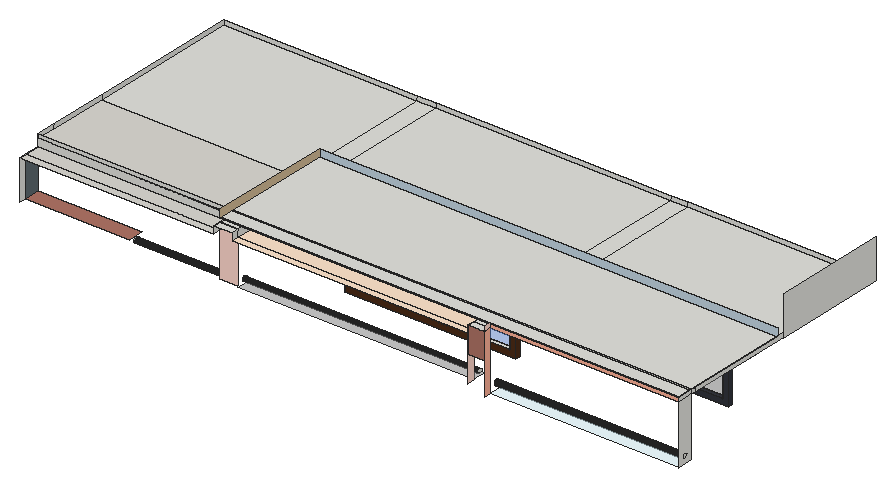
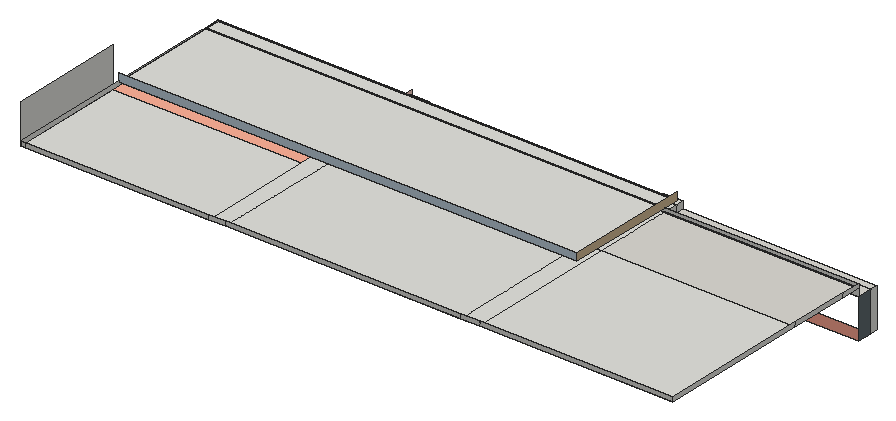
# SketchUp Ruby script. Lengths in inches.
U = 1.inch
M = Sketchup.active_model
def pt(a) = Geom::Point3d.new(a.map { |v| v * U })
def face(e, loops, mat)
  f = e.add_face(loops[0].map { |a| pt(a) })
  loops[1..].each { |l| e.add_face(l.map { |a| pt(a) }).erase! }
  f.material = f.back_material = mat if mat
  f
end
# faces: each face lists its corners as indices into pts; further lists are holes
def faces(e, pts, list, mat = nil) = list.each { |f| face(e, (f[0].is_a?(Array) ? f : [f]).map { |l| l.map { |i| pts[i] } }, mat) }
# xy, xz, yz: faces in a plane at the given z, y or x. An outline is a flat list of corners, or four numbers for a rectangle; further outlines are holes
def ring(l) = l.size == 4 ? [[l[0], l[1]], [l[2], l[1]], [l[2], l[3]], [l[0], l[3]]] : l.each_slice(2).to_a
def flat(e, list, mat, &to3) = list.each { |f| face(e, (f[0].is_a?(Array) ? f : [f]).map { |l| ring(l).map { |u, v| to3.(u, v) } }, mat) }
def xy(e, z, list, mat = nil) = flat(e, list, mat) { |x, y| [x, y, z] }
def xz(e, y, list, mat = nil) = flat(e, list, mat) { |x, z| [x, y, z] }
def yz(e, x, list, mat = nil) = flat(e, list, mat) { |y, z| [x, y, z] }
def lines(e, pts, list) = list.each { |a, b| e.add_line(pt(pts[a]), pt(pts[b])) }
# prism: a flat outline (further loops are holes) pulled along v
def prism(e, loops, v, mat = nil)
  f = face(e, loops, mat); d = Geom::Vector3d.new(v.map { |x| x * U })
  f.pushpull(f.normal.samedirection?(d) ? d.length : -d.length)
end
def box(e, o, s, mat = nil) = prism(e, [[o, [o[0] + s[0], o[1], o[2]], [o[0] + s[0], o[1] + s[1], o[2]], [o[0], o[1] + s[1], o[2]]]], [0, 0, s[2]], mat)
def at(x, y, z, deg = 0) = Geom::Transformation.translation(pt([x, y, z])) * Geom::Transformation.rotation(ORIGIN, Z_AXIS, deg.degrees)
def axes(o, x, y, z) = Geom::Transformation.new([*x, 0, *y, 0, *z, 0, *pt(o).to_a, 1])
def part(name) = M.definitions.add(name)
# library, detail: a bought-in or finely detailed component or shape, given as its bounding box
def library(name, o, s) = part(name).tap { |d| box(d.entities, o, s) }
def detail(e, o, s) = box(e.add_group.entities, o, s)
def put(e, d, t, mat = nil) = e.add_instance(d, t).tap { |i| i.material = mat if mat }
def group(e, t, mat = nil) = e.add_group.tap { |g| g.transformation = t; g.material = mat if mat }.entities
root = M.entities
M.materials.add("[Color B01]").color = [255, 216, 204]
M.materials.add("[Color B02]").color = [255, 178, 153]
M.materials.add("[Color C01]").color = [255, 229, 204]
M.materials.add("[Formica Beige]").color = [211, 187, 149]
M.materials.add("[Formica Graystone]").color = [149, 146, 135]
M.materials.add("[Formica Laminate Dark]").color = [50, 53, 60]
M.materials.add("[Formica Speckled Grey]").color = [94, 105, 111]
M.materials.add("[Stone Flagstone Ashlar]").color = [175, 116, 102]
M.materials.add("[Stone Flagstone Ashlar]1").color = [175, 116, 102]
M.materials.add("[Terrazzo Light Blue]").color = [196, 214, 227]
M.materials.add("[Terrazzo Tile Light]").color = [219, 217, 210]
M.materials.add("[Translucent Glass Blue]").color = [100, 149, 237]
M.materials["[Translucent Glass Blue]"].alpha = 0.5
M.materials.add("[Translucent Glass Gray]").color = [128, 128, 128]
M.materials["[Translucent Glass Gray]"].alpha = 0.5
M.materials.add("[Translucent Glass Safety]").color = [204, 235, 244]
M.materials["[Translucent Glass Safety]"].alpha = 0.5
M.materials.add("[Wood Veneer 01]").color = [76, 44, 23]
xy(root,2142.09,[[1358.7,1144.55,1824.89,1156.55]])
xy(root,2155.2,[[2073.08,1246.05,2321.89,1258.05]])
xy(root,2158.13,[[1374.73,1144.55,1482.83,1156.55],[1499.58,1144.55,1598.96,1156.55],[1615.7,1144.55,1695.53,1156.55],[1712.28,1144.55,1808.85,1156.55]])
xy(root,2169.37,[[2087.25,1246.05,2188.13,1258.05],[2208.5,1246.05,2307.73,1258.05]],"[Formica Laminate Dark]")
xy(root,2209.0625,[[1950.59,899.87,2463.34,941.93]],"[Translucent Glass Safety]")
xy(root,2226.5,[[1263.92,899.87,1905.54,941.93]],"[Translucent Glass Gray]")
xy(root,2228,[[1110.56,919.11,1111.89,919.29,1113.12,919.8,1114.18,920.61,1115,921.68,1115.51,922.91,1115.68,924.24,1115.51,925.57,1115,926.8,1114.18,927.86,1113.12,928.68,1111.89,929.1875,1110.56,929.36,1109.23,929.1875,1108,928.68,1106.94,927.86,1106.12,926.8,1105.61,925.57,1105.43,924.24,1105.61,922.91,1106.12,921.68,1106.94,920.61,1108,919.8,1109.23,919.29]])
xy(root,2230.84,[[982.87,919.11,984.2,919.29,985.43,919.8,986.5,920.61,987.31,921.68,987.82,922.91,988,924.24,987.82,925.57,987.31,926.8,986.78,927.49,978.96,927.49,978.43,926.8,977.92,925.57,977.75,924.24,977.92,922.91,978.43,921.68,979.25,920.61,980.31,919.8,981.55,919.29],[1021.75,919.11,1023.07,919.29,1024.31,919.8,1025.37,920.61,1026.18,921.68,1026.7,922.91,1026.87,924.24,1026.7,925.57,1026.18,926.8,1025.66,927.49,1017.84,927.49,1017.31,926.8,1016.8,925.57,1016.62,924.24,1016.8,922.91,1017.31,921.68,1018.12,920.61,1019.18,919.8,1020.42,919.29],[1060.43,919.11,1061.76,919.29,1063,919.8,1064.06,920.61,1064.87,921.68,1065.38,922.91,1065.56,924.24,1065.38,925.57,1064.87,926.8,1064.34,927.49,1056.53,927.49,1056,926.8,1055.48,925.57,1055.31,924.24,1055.48,922.91,1056,921.68,1056.81,920.61,1057.87,919.8,1059.11,919.29],[1156.68,919.11,1158.01,919.29,1159.25,919.8,1160.31,920.61,1161.12,921.68,1161.63,922.91,1161.81,924.24,1161.63,925.57,1161.12,926.8,1160.59,927.49,1152.78,927.49,1152.25,926.8,1151.73,925.57,1151.56,924.24,1151.73,922.91,1152.25,921.68,1153.06,920.61,1154.12,919.8,1155.36,919.29],[978.96,927.49,986.78,927.49,986.5,927.86,985.43,928.68,984.2,929.1875,982.87,929.36,981.55,929.1875,980.31,928.68,979.25,927.86],
  [1017.84,927.49,1025.66,927.49,1025.37,927.86,1024.31,928.68,1023.07,929.1875,1021.75,929.36,1020.42,929.1875,1019.18,928.68,1018.12,927.86],[1056.53,927.49,1064.34,927.49,1064.06,927.86,1063,928.68,1061.76,929.1875,1060.43,929.36,1059.11,929.1875,1057.87,928.68,1056.81,927.86],[1152.78,927.49,1160.59,927.49,1160.31,927.86,1159.25,928.68,1158.01,929.1875,1156.68,929.36,1155.36,929.1875,1154.12,928.68,1153.06,927.86]])
xy(root,2232,[[1197.43,919.11,1198.76,919.29,1200,919.8,1201.06,920.61,1201.87,921.68,1202.38,922.91,1202.56,924.24,1202.38,925.57,1201.87,926.8,1201.06,927.86,1200,928.68,1198.76,929.1875,1197.43,929.36,1196.11,929.1875,1194.87,928.68,1193.81,927.86,1193,926.8,1192.48,925.57,1192.31,924.24,1192.48,922.91,1193,921.68,1193.81,920.61,1194.87,919.8,1196.11,919.29]])
xy(root,2241,[[686.75,899.87,969.66,941.93]],"[Stone Flagstone Ashlar]")
xy(root,2326.25,[[1374.73,1144.55,1482.83,1156.55],[1499.58,1144.55,1598.96,1156.55],[1615.7,1144.55,1695.53,1156.55],[1712.28,1144.55,1808.85,1156.55]])
xy(root,2334.85,[[2087.25,1246.05,2188.13,1258.05],[2208.5,1246.05,2307.73,1258.05]],"[Formica Laminate Dark]")
xy(root,2342.28,[[1358.7,1144.55,1824.89,1156.55]])
xy(root,2349.01,[[2073.08,1246.05,2321.89,1258.05]])
xy(root,2350.0625,[[1263.92,880.68,1905.54,899.87],[1263.92,899.87,1905.54,941.93]],"[Color C01]")
xy(root,2350.0625,[[686.75,880.68,1214.63,899.87],[686.75,899.87,1214.63,941.93]],"[Terrazzo Tile Light]")
xy(root,2369.6875,[[1214.63,880.68,1263.92,899.87],[1905.54,880.68,1950.59,899.87],[1214.63,899.87,1263.92,941.93],[1905.54,899.87,1950.59,941.93],[1214.63,941.93,1263.92,1156.55],
  [1905.54,941.93,1950.59,1156.55],[686.75,1156.55,1214.63,1571.68],[1214.63,1156.55,1263.92,1571.68],[1263.92,1156.55,1905.54,1571.68],[1905.54,1156.55,1950.59,1571.68],
  [1950.59,1258.05,2463.34,1571.68],[2463.34,1258.05,2464.28,1571.68]])
xy(root,2369.6875,[[1950.59,899.87,2463.34,941.93],[1950.59,941.93,2463.34,1156.55],[1950.59,1156.55,2463.34,1258.05]],"[Color B02]")
xy(root,2369.6875,[[1263.92,941.93,1905.54,1156.55]],"[Color C01]")
xy(root,2369.6875,[[686.75,941.93,1214.63,1156.55]],"[Terrazzo Tile Light]")
xy(root,2379.45,[[1215.84,899.87,2463.34,1237.41]])
xz(root,880.68,[[1905.54,2298.64,1950.59,2369.6875]],"[Stone Flagstone Ashlar]1")
xz(root,899.87,[[1215.84,2379.45,1950.59,2381.6875]])
xz(root,899.87,[[1214.63,2230.66,1263.92,2369.6875],[1950.59,2379.45,2463.34,2381.6875]],"[Color B01]")
xz(root,899.87,[[1950.59,2369.6875,2463.34,2379.45]],"[Color B02]")
xz(root,941.93,[[686.75,2350.0625,1214.63,2369.6875],[1263.92,2350.0625,1905.54,2369.6875],[686.75,2369.6875,2463.34,2381.6875]])
xz(root,1144.55,[[[1358.7,2142.09,1824.89,2342.28],[1374.73,2158.13,1808.85,2326.25]],[1482.83,2158.13,1499.58,2326.25],[1598.96,2158.13,1615.7,2326.25],[1695.53,2158.13,1712.28,2326.25]],"[Wood Veneer 01]")
xz(root,1156.55,[[1374.73,2158.13,1482.83,2326.25],[1499.58,2158.13,1598.96,2326.25],[1615.7,2158.13,1695.53,2326.25],[1712.28,2158.13,1808.85,2326.25]],"[Translucent Glass Blue]")
xz(root,1237.41,[[1215.84,2379.45,2463.34,2400.95]],"[Terrazzo Light Blue]")
xz(root,1246.05,[[[2073.08,2155.2,2321.89,2349.01],[2087.25,2169.37,2307.73,2334.85]],[2188.13,2169.37,2208.5,2334.85]],"[Formica Laminate Dark]")
xz(root,1258.05,[[2087.25,2169.37,2188.13,2334.85],[2208.5,2169.37,2307.73,2334.85]],"[Translucent Glass Gray]")
xz(root,1571.68,[[686.75,2369.6875,1214.63,2381.6875],[1214.63,2369.6875,1263.92,2381.6875],[1263.92,2369.6875,1905.54,2381.6875],[1905.54,2369.6875,1950.59,2381.6875],[1950.59,2369.6875,2448.8,2381.6875],
  [2448.8,2369.6875,2463.34,2381.6875],[2463.34,2369.6875,2464.28,2476.875]])
yz(root,686.75,[[880.68,2241,899.87,2350.0625],[941.93,2369.6875,994.87,2381.6875],[994.87,2369.6875,1156.55,2381.6875],[1156.55,2369.6875,1571.68,2381.6875]])
yz(root,686.75,[[899.87,2241,941.93,2350.0625]],"[Formica Speckled Grey]")
yz(root,969.66,[[921.12,2224.46,919.47,2224.68,917.93,2225.3125,916.61,2226.33,915.6,2227.65,914.96,2229.19,914.74,2230.84,914.96,2232.49,915.6,2234.02,916.61,2235.34,917.93,2236.36,919.47,2236.99,921.12,2237.21,922.77,2236.99,924.3,2236.36,925.625,2235.34,926.64,2234.02,927.27,2232.49,927.49,2230.84,927.27,2229.19,926.64,2227.65,925.625,2226.33,924.3,2225.3125,922.77,2224.68]])
yz(root,1214.63,[[880.68,2350.0625,899.87,2369.6875],[899.87,2350.0625,941.93,2369.6875]])
yz(root,1215.84,[[899.87,2379.45,1237.41,2400.95]],"[Formica Beige]")
yz(root,1263.92,[[880.68,2350.0625,899.87,2369.6875],[899.87,2350.0625,941.93,2369.6875]])
yz(root,1358.7,[[1144.55,2142.09,1156.55,2342.28]],"[Wood Veneer 01]")
yz(root,1374.73,[[1144.55,2158.13,1156.55,2326.25]],"[Wood Veneer 01]")
yz(root,1482.83,[[1144.55,2158.13,1156.55,2326.25]],"[Wood Veneer 01]")
yz(root,1499.58,[[1144.55,2158.13,1156.55,2326.25]],"[Wood Veneer 01]")
yz(root,1598.96,[[1144.55,2158.13,1156.55,2326.25]],"[Wood Veneer 01]")
yz(root,1615.7,[[1144.55,2158.13,1156.55,2326.25]],"[Wood Veneer 01]")
yz(root,1695.53,[[1144.55,2158.13,1156.55,2326.25]],"[Wood Veneer 01]")
yz(root,1712.28,[[1144.55,2158.13,1156.55,2326.25]],"[Wood Veneer 01]")
yz(root,1808.85,[[1144.55,2158.13,1156.55,2326.25]],"[Wood Veneer 01]")
yz(root,1824.89,[[1144.55,2142.09,1156.55,2342.28]],"[Wood Veneer 01]")
yz(root,1905.54,[[920.9,2234.39,922.34,2234.58,923.68,2235.14,924.83,2236.02,925.72,2237.18,926.27,2238.52,926.46,2239.96,926.27,2241.4,925.72,2242.74,924.83,2243.89,923.68,2244.77,922.34,2245.33,920.9,2245.52,919.46,2245.33,918.12,2244.77,916.97,2243.89,916.08,2242.74,915.53,2241.4,915.34,2239.96,915.53,2238.52,916.08,2237.18,916.97,2236.02,918.12,2235.14,919.46,2234.58],[880.68,2350.0625,899.87,2369.6875],[899.87,2350.0625,941.93,2369.6875]])
yz(root,1905.54,[[880.68,2226.5,899.87,2350.0625]],"[Color B01]")
yz(root,1950.59,[[880.68,2369.6875,899.87,2383.06]],"[Color B01]")
yz(root,1950.59,[[880.68,2209.0625,899.87,2369.6875]],"[Color B02]")
yz(root,2073.08,[[1246.05,2155.2,1258.05,2349.01]],"[Formica Laminate Dark]")
yz(root,2087.25,[[1246.05,2169.37,1258.05,2334.85]],"[Formica Laminate Dark]")
yz(root,2188.13,[[1246.05,2169.37,1258.05,2334.85]],"[Formica Laminate Dark]")
yz(root,2208.5,[[1246.05,2169.37,1258.05,2334.85]],"[Formica Laminate Dark]")
yz(root,2307.73,[[1246.05,2169.37,1258.05,2334.85]],"[Formica Laminate Dark]")
yz(root,2321.89,[[1246.05,2155.2,1258.05,2349.01]],"[Formica Laminate Dark]")
yz(root,2463.34,[[[899.87,2209.0625,941.93,2369.6875],[920.9,2220.96,922.7,2221.2,924.37,2221.89,925.81,2222.99,926.91,2224.43,927.6,2226.1,927.84,2227.9,927.6,2229.69,926.91,2231.37,925.81,2232.8,924.37,2233.91,922.7,2234.6,920.9,2234.84,919.11,2234.6,917.43,2233.91,916,2232.8,914.89,2231.37,914.2,2229.69,913.96,2227.9,914.2,2226.1,914.89,2224.43,916,2222.99,917.43,2221.89,919.11,2221.2]],[920.9,2220.96,922.7,2221.2,924.37,2221.89,925.81,2222.99,926.91,2224.43,927.6,2226.1,927.84,2227.9,927.6,2229.69,926.91,2231.37,925.81,2232.8,924.37,2233.91,922.7,2234.6,920.9,2234.84,919.11,2234.6,917.43,2233.91,916,2232.8,914.89,2231.37,914.2,2229.69,913.96,2227.9,914.2,2226.1,914.89,2224.43,916,2222.99,917.43,2221.89,919.11,2221.2],[899.87,2369.6875,941.93,2379.45],[941.93,2369.6875,954.56,2379.45],[954.56,2369.6875,1571.68,2369.6875,1571.68,2381.6875,1237.41,2381.6875,1237.41,2379.45,954.56,2379.45],
  [899.87,2379.45,941.93,2381.6875],[941.93,2379.45,952.49,2381.6875],[952.49,2379.45,954.56,2381.6875],[954.56,2379.45,1237.41,2381.6875]])
yz(root,2464.28,[[1258.05,2369.6875,1571.68,2476.875]])
p = [[2463.34,920.9,2220.96],[2463.34,919.11,2221.2],[1950.59,919.11,2221.2],[1950.59,920.9,2220.96],[2463.34,922.7,2221.2],[1950.59,922.7,2221.2],
  [2463.34,917.43,2221.89],[1950.59,917.43,2221.89],[2463.34,924.37,2221.89],[1950.59,924.37,2221.89],[2463.34,916,2222.99],[1950.59,916,2222.99],
  [2463.34,925.81,2222.99],[1950.59,925.81,2222.99],[2463.34,914.89,2224.43],[1950.59,914.89,2224.43],[2463.34,926.91,2224.43],[1950.59,926.91,2224.43],
  [2463.34,914.2,2226.1],[1950.59,914.2,2226.1],[2463.34,927.6,2226.1],[1950.59,927.6,2226.1],[969.66,919.47,2224.68],[969.66,921.12,2224.46],
  [1214.63,921.12,2224.46],[1214.63,919.47,2224.68],[969.66,922.77,2224.68],[1214.63,922.77,2224.68],[969.66,917.93,2225.3125],[1214.63,917.93,2225.3125],
  [969.66,924.3,2225.3125],[1214.63,924.3,2225.3125],[969.66,916.61,2226.33],[1214.63,916.61,2226.33],[969.66,925.625,2226.33],[1214.63,925.625,2226.33],
  [2463.34,913.96,2227.9],[1950.59,913.96,2227.9],[2463.34,927.84,2227.9],[1950.59,927.84,2227.9],[969.66,915.6,2227.65],[1214.63,915.6,2227.65],
  [969.66,926.64,2227.65],[1214.63,926.64,2227.65],[969.66,914.96,2229.19],[1214.63,914.96,2229.19],[969.66,927.27,2229.19],[1214.63,927.27,2229.19],
  [2463.34,914.2,2229.69],[1950.59,914.2,2229.69],[2463.34,927.6,2229.69],[1950.59,927.6,2229.69],[969.66,914.74,2230.84],[1214.63,914.74,2230.84],
  [969.66,927.49,2230.84],[978.96,927.49,2230.84],[986.78,927.49,2230.84],[1017.84,927.49,2230.84],[1025.66,927.49,2230.84],[1056.53,927.49,2230.84],
  [1064.34,927.49,2230.84],[1152.78,927.49,2230.84],[1160.59,927.49,2230.84],[1214.63,927.49,2230.84],[2463.34,914.89,2231.37],[1950.59,914.89,2231.37],
  [2463.34,926.91,2231.37],[1950.59,926.91,2231.37],[969.66,914.96,2232.49],[1214.63,914.96,2232.49],[969.66,927.27,2232.49],[1214.63,927.27,2232.49],
  [2463.34,916,2232.8],[1950.59,916,2232.8],[2463.34,925.81,2232.8],[1950.59,925.81,2232.8],[969.66,915.6,2234.02],[1214.63,915.6,2234.02],
  [969.66,926.64,2234.02],[1214.63,926.64,2234.02],[2463.34,917.43,2233.91],[1950.59,917.43,2233.91],[2463.34,924.37,2233.91],[1950.59,924.37,2233.91],
  [2463.34,919.11,2234.6],[1950.59,919.11,2234.6],[2463.34,922.7,2234.6],[1950.59,922.7,2234.6],[969.66,916.61,2235.34],[1214.63,916.61,2235.34],
  [969.66,925.625,2235.34],[1214.63,925.625,2235.34],[1905.54,920.9,2234.39],[1905.54,919.46,2234.58],[1263.92,919.46,2234.58],[1263.92,920.9,2234.39],
  [1905.54,922.34,2234.58],[1263.92,922.34,2234.58],[1905.54,918.12,2235.14],[1263.92,918.12,2235.14],[2463.34,920.9,2234.84],[1950.59,920.9,2234.84],
  [1905.54,923.68,2235.14],[1263.92,923.68,2235.14],[1905.54,916.97,2236.02],[1263.92,916.97,2236.02],[1905.54,924.83,2236.02],[1263.92,924.83,2236.02],
  [969.66,917.93,2236.36],[1214.63,917.93,2236.36],[969.66,924.3,2236.36],[1214.63,924.3,2236.36],[1905.54,916.08,2237.18],[1263.92,916.08,2237.18],
  [1905.54,925.72,2237.18],[1263.92,925.72,2237.18],[969.66,919.47,2236.99],[1214.63,919.47,2236.99],[969.66,922.77,2236.99],[1214.63,922.77,2236.99],
  [969.66,921.12,2237.21],[1214.63,921.12,2237.21],[1905.54,915.53,2238.52],[1263.92,915.53,2238.52],[1905.54,926.27,2238.52],[1263.92,926.27,2238.52],
  [1905.54,915.34,2239.96],[1263.92,915.34,2239.96],[1905.54,926.46,2239.96],[1263.92,926.46,2239.96],[1905.54,915.53,2241.4],[1263.92,915.53,2241.4],
  [1905.54,926.27,2241.4],[1263.92,926.27,2241.4],[1905.54,916.08,2242.74],[1263.92,916.08,2242.74],[1905.54,925.72,2242.74],[1263.92,925.72,2242.74],
  [1905.54,916.97,2243.89],[1263.92,916.97,2243.89],[1905.54,924.83,2243.89],[1263.92,924.83,2243.89],[1905.54,918.12,2244.77],[1263.92,918.12,2244.77],
  [1905.54,923.68,2244.77],[1263.92,923.68,2244.77],[1905.54,919.46,2245.33],[1263.92,919.46,2245.33],[1905.54,922.34,2245.33],[1263.92,922.34,2245.33],
  [1905.54,920.9,2245.52],[1263.92,920.9,2245.52]]
faces(root,p,[[0,1,2,3],[4,0,3,5],[1,6,7,2],[8,4,5,9],[6,10,11,7],[12,8,9,13],[10,14,15,11],[16,12,13,17],
  [14,18,19,15],[20,16,17,21],[18,36,37,19],[38,20,21,39],[36,48,49,37],[50,38,39,51],[48,64,65,49],[66,50,51,67],
  [64,72,73,65],[74,66,67,75],[72,80,81,73],[82,74,75,83],[80,84,85,81],[86,82,83,87],[92,93,94,95],[96,92,95,97],
  [93,98,99,94],[84,100,101,85],[100,86,87,101],[102,96,97,103],[98,104,105,99],[106,102,103,107],[104,112,113,105],[114,106,107,115],
  [112,122,123,113],[124,114,115,125],[122,126,127,123],[128,124,125,129],[126,130,131,127],[132,128,129,133],[130,134,135,131],[136,132,133,137],
  [134,138,139,135],[140,136,137,141],[138,142,143,139],[144,140,141,145],[142,146,147,143],[148,144,145,149],[146,150,151,147],[150,148,149,151]],"[Formica Laminate Dark]")
faces(root,p,[[22,23,24,25],[23,26,27,24],[28,22,25,29],[26,30,31,27],[32,28,29,33],[30,34,35,31],[40,32,33,41],[34,42,43,35],
  [44,40,41,45],[42,46,47,43],[52,44,45,53],[46,54,55,56,57,58,59,60,61,62,63,47],[68,52,53,69],[54,70,71,63,62,61,60,59,58,57,56,55],[76,68,69,77],[70,78,79,71],
  [88,76,77,89],[78,90,91,79],[108,88,89,109],[90,110,111,91],[116,108,109,117],[110,118,119,111],[120,116,117,121],[118,120,121,119]],"[Formica Graystone]")
